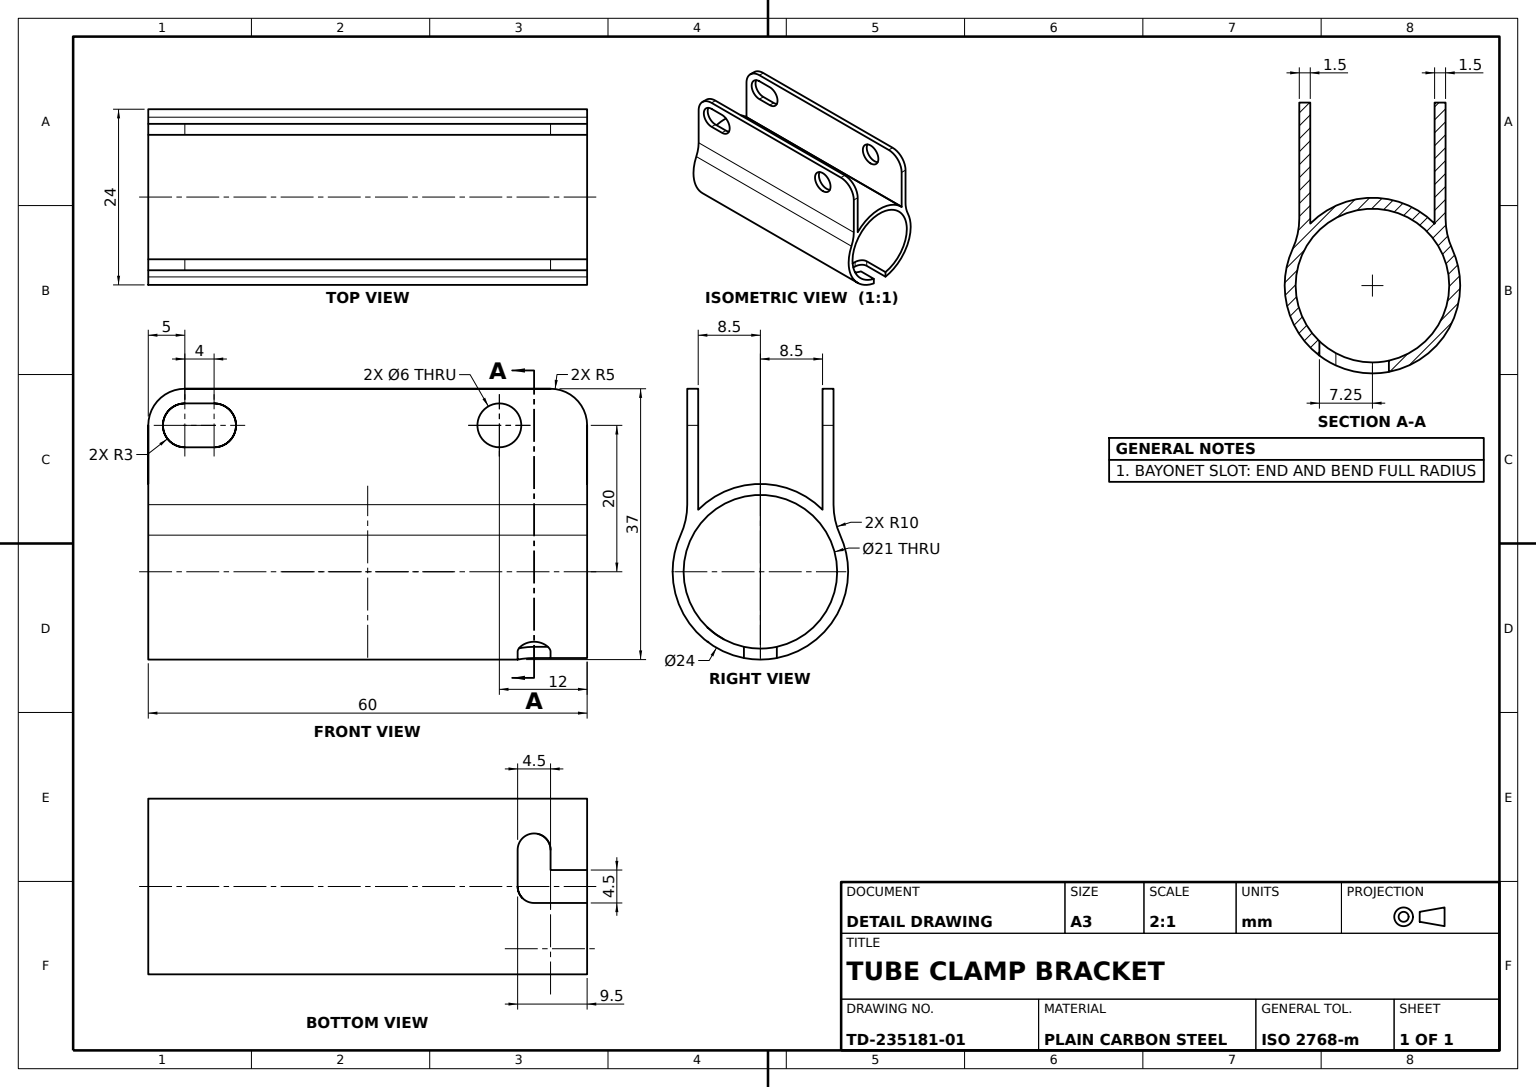
ISO-10303-21;
HEADER;
FILE_DESCRIPTION((''),'2;1');
FILE_NAME('','',(''),(''),'','','');
FILE_SCHEMA(('AUTOMOTIVE_DESIGN'));
ENDSEC;
DATA;
#1=APPLICATION_CONTEXT('');
#2=PRODUCT_CONTEXT('',#1,'mechanical');
#3=PRODUCT('','','',(#2));
#4=PRODUCT_DEFINITION_FORMATION('','',#3);
#5=PRODUCT_DEFINITION_CONTEXT('',#1,'design');
#6=PRODUCT_DEFINITION('','',#4,#5);
#7=PRODUCT_DEFINITION_SHAPE('','',#6);
#8=(LENGTH_UNIT()NAMED_UNIT(*)SI_UNIT(.MILLI.,.METRE.));
#9=(NAMED_UNIT(*)PLANE_ANGLE_UNIT()SI_UNIT($,.RADIAN.));
#10=(NAMED_UNIT(*)SI_UNIT($,.STERADIAN.)SOLID_ANGLE_UNIT());
#11=UNCERTAINTY_MEASURE_WITH_UNIT(LENGTH_MEASURE(1.E-05),#8,'distance_accuracy_value','');
#12=(GEOMETRIC_REPRESENTATION_CONTEXT(3)GLOBAL_UNCERTAINTY_ASSIGNED_CONTEXT((#11))GLOBAL_UNIT_ASSIGNED_CONTEXT((#8,#9,#10))REPRESENTATION_CONTEXT('',''));
#13=CARTESIAN_POINT('',(-10.909091,4.999173,30.));
#14=VERTEX_POINT('',#13);
#15=CARTESIAN_POINT('',(-10.909091,4.999173,-30.));
#16=VERTEX_POINT('',#15);
#17=DIRECTION('',(0.,0.,-1.));
#18=VECTOR('',#17,1000.);
#19=LINE('',#13,#18);
#20=EDGE_CURVE('',#14,#16,#19,.T.);
#21=ORIENTED_EDGE('',*,*,#20,.T.);
#22=CARTESIAN_POINT('',(-12.,0.,-30.));
#23=VERTEX_POINT('',#22);
#24=CARTESIAN_POINT('',(0.,0.,-30.));
#25=DIRECTION('',(0.,0.,1.));
#26=DIRECTION('',(1.,0.,0.));
#27=AXIS2_PLACEMENT_3D('',#24,#25,#26);
#28=CIRCLE('',#27,12.);
#29=EDGE_CURVE('',#16,#23,#28,.T.);
#30=ORIENTED_EDGE('',*,*,#29,.T.);
#31=CARTESIAN_POINT('',(-12.,0.,30.));
#32=VERTEX_POINT('',#31);
#33=LINE('',#31,#18);
#34=EDGE_CURVE('',#32,#23,#33,.T.);
#35=ORIENTED_EDGE('',*,*,#34,.F.);
#36=CARTESIAN_POINT('',(0.,0.,30.));
#37=AXIS2_PLACEMENT_3D('',#36,#25,#26);
#38=CIRCLE('',#37,12.);
#39=EDGE_CURVE('',#14,#32,#38,.T.);
#40=ORIENTED_EDGE('',*,*,#39,.F.);
#41=EDGE_LOOP('',(#21,#30,#35,#40));
#42=FACE_OUTER_BOUND('',#41,.T.);
#43=DIRECTION('',(-1.,0.,0.));
#44=AXIS2_PLACEMENT_3D('',#36,#17,#43);
#45=CYLINDRICAL_SURFACE('',#44,12.);
#46=ADVANCED_FACE('',(#42),#45,.T.);
#47=CARTESIAN_POINT('',(-2.25,-10.256096,-30.));
#48=VERTEX_POINT('',#47);
#49=CARTESIAN_POINT('',(-2.25,-10.256096,-22.75));
#50=VERTEX_POINT('',#49);
#51=CARTESIAN_POINT('',(-2.25,-10.256096,30.));
#52=VECTOR('',#25,1000.);
#53=LINE('',#51,#52);
#54=EDGE_CURVE('',#48,#50,#53,.T.);
#55=ORIENTED_EDGE('',*,*,#54,.T.);
#56=CARTESIAN_POINT('',(-2.25,-11.787175,-22.75));
#57=VERTEX_POINT('',#56);
#58=CARTESIAN_POINT('',(-2.25,-12.001,-22.75));
#59=DIRECTION('',(0.,1.,0.));
#60=VECTOR('',#59,1000.);
#61=LINE('',#58,#60);
#62=EDGE_CURVE('',#57,#50,#61,.T.);
#63=ORIENTED_EDGE('',*,*,#62,.F.);
#64=CARTESIAN_POINT('',(-2.25,-11.787175,-30.));
#65=VERTEX_POINT('',#64);
#66=CARTESIAN_POINT('',(-2.25,-11.787175,30.));
#67=LINE('',#66,#18);
#68=EDGE_CURVE('',#57,#65,#67,.T.);
#69=ORIENTED_EDGE('',*,*,#68,.T.);
#70=CARTESIAN_POINT('',(-2.25,-12.001,-30.));
#71=LINE('',#70,#60);
#72=EDGE_CURVE('',#65,#48,#71,.T.);
#73=ORIENTED_EDGE('',*,*,#72,.T.);
#74=EDGE_LOOP('',(#55,#63,#69,#73));
#75=FACE_OUTER_BOUND('',#74,.T.);
#76=AXIS2_PLACEMENT_3D('',#70,#43,#25);
#77=PLANE('',#76);
#78=ADVANCED_FACE('',(#75),#77,.F.);
#79=CARTESIAN_POINT('',(10.909091,4.999173,30.));
#80=VERTEX_POINT('',#79);
#81=CARTESIAN_POINT('',(10.,9.165151,30.));
#82=VERTEX_POINT('',#81);
#83=CARTESIAN_POINT('',(20.,9.165151,30.));
#84=AXIS2_PLACEMENT_3D('',#83,#17,#26);
#85=CIRCLE('',#84,10.);
#86=EDGE_CURVE('',#80,#82,#85,.T.);
#87=ORIENTED_EDGE('',*,*,#86,.F.);
#88=CARTESIAN_POINT('',(10.909091,4.999173,-30.));
#89=VERTEX_POINT('',#88);
#90=LINE('',#79,#52);
#91=EDGE_CURVE('',#89,#80,#90,.T.);
#92=ORIENTED_EDGE('',*,*,#91,.F.);
#93=CARTESIAN_POINT('',(10.,9.165151,-30.));
#94=VERTEX_POINT('',#93);
#95=CARTESIAN_POINT('',(20.,9.165151,-30.));
#96=AXIS2_PLACEMENT_3D('',#95,#25,#26);
#97=CIRCLE('',#96,10.);
#98=EDGE_CURVE('',#94,#89,#97,.T.);
#99=ORIENTED_EDGE('',*,*,#98,.F.);
#100=LINE('',#93,#18);
#101=EDGE_CURVE('',#82,#94,#100,.T.);
#102=ORIENTED_EDGE('',*,*,#101,.F.);
#103=EDGE_LOOP('',(#87,#92,#99,#102));
#104=FACE_OUTER_BOUND('',#103,.T.);
#105=AXIS2_PLACEMENT_3D('',#83,#17,#43);
#106=CYLINDRICAL_SURFACE('',#105,10.);
#107=ADVANCED_FACE('',(#104),#106,.F.);
#108=CARTESIAN_POINT('',(12.,0.,30.));
#109=VERTEX_POINT('',#108);
#110=EDGE_CURVE('',#109,#80,#38,.T.);
#111=ORIENTED_EDGE('',*,*,#110,.F.);
#112=CARTESIAN_POINT('',(12.,0.,-30.));
#113=VERTEX_POINT('',#112);
#114=LINE('',#108,#18);
#115=EDGE_CURVE('',#109,#113,#114,.T.);
#116=ORIENTED_EDGE('',*,*,#115,.T.);
#117=EDGE_CURVE('',#113,#89,#28,.T.);
#118=ORIENTED_EDGE('',*,*,#117,.T.);
#119=ORIENTED_EDGE('',*,*,#91,.T.);
#120=EDGE_LOOP('',(#111,#116,#118,#119));
#121=FACE_OUTER_BOUND('',#120,.T.);
#122=ADVANCED_FACE('',(#121),#45,.T.);
#123=CARTESIAN_POINT('',(2.25,-11.787175,-25.));
#124=VERTEX_POINT('',#123);
#125=CARTESIAN_POINT('',(5.,-10.908712,-25.));
#126=VERTEX_POINT('',#125);
#127=CARTESIAN_POINT('',(0.,0.,-25.));
#128=AXIS2_PLACEMENT_3D('',#127,#25,#43);
#129=CIRCLE('',#128,12.);
#130=EDGE_CURVE('',#124,#126,#129,.T.);
#131=ORIENTED_EDGE('',*,*,#130,.F.);
#132=CARTESIAN_POINT('',(2.25,-11.787175,-30.));
#133=VERTEX_POINT('',#132);
#134=CARTESIAN_POINT('',(2.25,-11.787175,30.));
#135=LINE('',#134,#52);
#136=EDGE_CURVE('',#133,#124,#135,.T.);
#137=ORIENTED_EDGE('',*,*,#136,.F.);
#138=EDGE_CURVE('',#133,#113,#28,.T.);
#139=ORIENTED_EDGE('',*,*,#138,.T.);
#140=ORIENTED_EDGE('',*,*,#115,.F.);
#141=EDGE_CURVE('',#32,#109,#38,.T.);
#142=ORIENTED_EDGE('',*,*,#141,.F.);
#143=ORIENTED_EDGE('',*,*,#34,.T.);
#144=EDGE_CURVE('',#23,#65,#28,.T.);
#145=ORIENTED_EDGE('',*,*,#144,.T.);
#146=ORIENTED_EDGE('',*,*,#68,.F.);
#147=CARTESIAN_POINT('',(0.,-12.,-20.5));
#148=VERTEX_POINT('',#147);
#149=CARTESIAN_POINT('',(-0.148916,-12.,-20.5));
#150=CARTESIAN_POINT('',(-0.29528,-11.997231,-20.514638));
#151=CARTESIAN_POINT('',(-0.583133,-11.986688,-20.571929));
#152=CARTESIAN_POINT('',(-0.726135,-11.978787,-20.615301));
#153=CARTESIAN_POINT('',(-0.998336,-11.959178,-20.728234));
#154=CARTESIAN_POINT('',(-1.127389,-11.947555,-20.797295));
#155=CARTESIAN_POINT('',(-1.371629,-11.921984,-20.960392));
#156=CARTESIAN_POINT('',(-1.487027,-11.907966,-21.055107));
#157=CARTESIAN_POINT('',(-1.797526,-11.866445,-21.365425));
#158=CARTESIAN_POINT('',(-1.965077,-11.83856,-21.615671));
#159=CARTESIAN_POINT('',(-2.189941,-11.799033,-22.156375));
#160=CARTESIAN_POINT('',(-2.25,-11.787175,-22.452172));
#161=B_SPLINE_CURVE_WITH_KNOTS('',3,(#147,#149,#150,#151,#152,#153,#154,#155,#156,#157,#158,#159,#160,#56),.UNSPECIFIED.,.F.,.F.,(4,2,2,2,2,2,4),(0.,0.000440334,0.000880667,0.001321001,0.001761334,0.002642001,0.003522668),.UNSPECIFIED.);
#162=EDGE_CURVE('',#148,#57,#161,.T.);
#163=ORIENTED_EDGE('',*,*,#162,.F.);
#164=CARTESIAN_POINT('',(5.,-10.908712,-20.5));
#165=VERTEX_POINT('',#164);
#166=CARTESIAN_POINT('',(0.,0.,-20.5));
#167=AXIS2_PLACEMENT_3D('',#166,#17,#26);
#168=CIRCLE('',#167,12.);
#169=EDGE_CURVE('',#165,#148,#168,.T.);
#170=ORIENTED_EDGE('',*,*,#169,.F.);
#171=CARTESIAN_POINT('',(5.291277,-10.775206,-25.));
#172=CARTESIAN_POINT('',(5.568793,-10.633901,-24.945399));
#173=CARTESIAN_POINT('',(6.096925,-10.340155,-24.734958));
#174=CARTESIAN_POINT('',(6.334777,-10.194776,-24.584238));
#175=CARTESIAN_POINT('',(6.755082,-9.921277,-24.187271));
#176=CARTESIAN_POINT('',(6.927005,-9.800041,-23.951534));
#177=CARTESIAN_POINT('',(7.115788,-9.662899,-23.530752));
#178=CARTESIAN_POINT('',(7.164502,-9.626613,-23.384151));
#179=CARTESIAN_POINT('',(7.23166,-9.576265,-23.076973));
#180=CARTESIAN_POINT('',(7.24941,-9.562743,-22.916453));
#181=CARTESIAN_POINT('',(7.250561,-9.561871,-22.599906));
#182=CARTESIAN_POINT('',(7.233989,-9.5745,-22.439219));
#183=CARTESIAN_POINT('',(7.168929,-9.623311,-22.131097));
#184=CARTESIAN_POINT('',(7.120922,-9.659108,-21.983251));
#185=CARTESIAN_POINT('',(6.996677,-9.749482,-21.701433));
#186=CARTESIAN_POINT('',(6.922276,-9.8027,-21.571326));
#187=CARTESIAN_POINT('',(6.751271,-9.921248,-21.329625));
#188=CARTESIAN_POINT('',(6.654513,-9.986635,-21.218426));
#189=CARTESIAN_POINT('',(6.342224,-10.19009,-20.921485));
#190=CARTESIAN_POINT('',(6.098757,-10.338984,-20.766451));
#191=CARTESIAN_POINT('',(5.576237,-10.629911,-20.5569));
#192=CARTESIAN_POINT('',(5.291702,-10.775011,-20.5));
#193=B_SPLINE_CURVE_WITH_KNOTS('',3,(#125,#171,#172,#173,#174,#175,#176,#177,#178,#179,#180,#181,#182,#183,#184,#185,#186,#187,#188,#189,#190,#191,#192,#164),.UNSPECIFIED.,.F.,.F.,(4,2,2,2,2,2,2,2,2,2,2,4),(0.,0.000947115,0.001894231,0.002841346,0.003314904,0.003788462,0.004262019,0.004735577,0.005209135,0.005682693,0.006629808,0.007576923),.UNSPECIFIED.);
#194=EDGE_CURVE('',#126,#165,#193,.T.);
#195=ORIENTED_EDGE('',*,*,#194,.F.);
#196=EDGE_LOOP('',(#131,#137,#139,#140,#142,#143,#145,#146,#163,#170,#195));
#197=FACE_OUTER_BOUND('',#196,.T.);
#198=ADVANCED_FACE('',(#197),#45,.T.);
#199=CARTESIAN_POINT('',(-10.,20.,-30.));
#200=VERTEX_POINT('',#199);
#201=CARTESIAN_POINT('',(-8.5,20.,-30.));
#202=VERTEX_POINT('',#201);
#203=VECTOR('',#26,1000.);
#204=LINE('',#201,#203);
#205=EDGE_CURVE('',#200,#202,#204,.T.);
#206=ORIENTED_EDGE('',*,*,#205,.F.);
#207=CARTESIAN_POINT('',(-10.,25.,-25.));
#208=VERTEX_POINT('',#207);
#209=CARTESIAN_POINT('',(-10.,20.,-25.));
#210=DIRECTION('',(0.,-1.,0.));
#211=AXIS2_PLACEMENT_3D('',#209,#43,#210);
#212=CIRCLE('',#211,5.);
#213=EDGE_CURVE('',#208,#200,#212,.T.);
#214=ORIENTED_EDGE('',*,*,#213,.F.);
#215=CARTESIAN_POINT('',(-8.5,25.,-25.));
#216=VERTEX_POINT('',#215);
#217=VECTOR('',#43,1000.);
#218=LINE('',#207,#217);
#219=EDGE_CURVE('',#216,#208,#218,.T.);
#220=ORIENTED_EDGE('',*,*,#219,.F.);
#221=CARTESIAN_POINT('',(-8.5,20.,-25.));
#222=AXIS2_PLACEMENT_3D('',#221,#26,#59);
#223=CIRCLE('',#222,5.);
#224=EDGE_CURVE('',#202,#216,#223,.T.);
#225=ORIENTED_EDGE('',*,*,#224,.F.);
#226=EDGE_LOOP('',(#206,#214,#220,#225));
#227=FACE_OUTER_BOUND('',#226,.T.);
#228=AXIS2_PLACEMENT_3D('',#209,#26,#17);
#229=CYLINDRICAL_SURFACE('',#228,5.);
#230=ADVANCED_FACE('',(#227),#229,.T.);
#231=CARTESIAN_POINT('',(8.5,20.,-30.));
#232=VERTEX_POINT('',#231);
#233=CARTESIAN_POINT('',(10.,20.,-30.));
#234=VERTEX_POINT('',#233);
#235=LINE('',#233,#203);
#236=EDGE_CURVE('',#232,#234,#235,.T.);
#237=ORIENTED_EDGE('',*,*,#236,.F.);
#238=CARTESIAN_POINT('',(8.5,25.,-25.));
#239=VERTEX_POINT('',#238);
#240=CARTESIAN_POINT('',(8.5,20.,-25.));
#241=AXIS2_PLACEMENT_3D('',#240,#43,#210);
#242=CIRCLE('',#241,5.);
#243=EDGE_CURVE('',#239,#232,#242,.T.);
#244=ORIENTED_EDGE('',*,*,#243,.F.);
#245=CARTESIAN_POINT('',(10.,25.,-25.));
#246=VERTEX_POINT('',#245);
#247=LINE('',#238,#217);
#248=EDGE_CURVE('',#246,#239,#247,.T.);
#249=ORIENTED_EDGE('',*,*,#248,.F.);
#250=CARTESIAN_POINT('',(10.,20.,-25.));
#251=AXIS2_PLACEMENT_3D('',#250,#26,#59);
#252=CIRCLE('',#251,5.);
#253=EDGE_CURVE('',#234,#246,#252,.T.);
#254=ORIENTED_EDGE('',*,*,#253,.F.);
#255=EDGE_LOOP('',(#237,#244,#249,#254));
#256=FACE_OUTER_BOUND('',#255,.T.);
#257=AXIS2_PLACEMENT_3D('',#250,#26,#17);
#258=CYLINDRICAL_SURFACE('',#257,5.);
#259=ADVANCED_FACE('',(#256),#258,.T.);
#260=CARTESIAN_POINT('',(-10.,9.165151,-30.));
#261=VERTEX_POINT('',#260);
#262=CARTESIAN_POINT('',(-10.,9.165151,30.));
#263=VERTEX_POINT('',#262);
#264=LINE('',#260,#52);
#265=EDGE_CURVE('',#261,#263,#264,.T.);
#266=ORIENTED_EDGE('',*,*,#265,.F.);
#267=CARTESIAN_POINT('',(-20.,9.165151,-30.));
#268=AXIS2_PLACEMENT_3D('',#267,#25,#26);
#269=CIRCLE('',#268,10.);
#270=EDGE_CURVE('',#16,#261,#269,.T.);
#271=ORIENTED_EDGE('',*,*,#270,.F.);
#272=ORIENTED_EDGE('',*,*,#20,.F.);
#273=CARTESIAN_POINT('',(-20.,9.165151,30.));
#274=AXIS2_PLACEMENT_3D('',#273,#17,#26);
#275=CIRCLE('',#274,10.);
#276=EDGE_CURVE('',#263,#14,#275,.T.);
#277=ORIENTED_EDGE('',*,*,#276,.F.);
#278=EDGE_LOOP('',(#266,#271,#272,#277));
#279=FACE_OUTER_BOUND('',#278,.T.);
#280=AXIS2_PLACEMENT_3D('',#273,#17,#43);
#281=CYLINDRICAL_SURFACE('',#280,10.);
#282=ADVANCED_FACE('',(#279),#281,.F.);
#283=CARTESIAN_POINT('',(5.,-9.233093,-20.5));
#284=VERTEX_POINT('',#283);
#285=CARTESIAN_POINT('',(5.,-12.001,-20.5));
#286=LINE('',#285,#60);
#287=EDGE_CURVE('',#165,#284,#286,.T.);
#288=ORIENTED_EDGE('',*,*,#287,.F.);
#289=ORIENTED_EDGE('',*,*,#169,.T.);
#290=CARTESIAN_POINT('',(0.,-10.5,-20.5));
#291=VERTEX_POINT('',#290);
#292=CARTESIAN_POINT('',(0.,-12.001,-20.5));
#293=LINE('',#292,#60);
#294=EDGE_CURVE('',#148,#291,#293,.T.);
#295=ORIENTED_EDGE('',*,*,#294,.T.);
#296=AXIS2_PLACEMENT_3D('',#166,#25,#26);
#297=CIRCLE('',#296,10.5);
#298=EDGE_CURVE('',#291,#284,#297,.T.);
#299=ORIENTED_EDGE('',*,*,#298,.T.);
#300=EDGE_LOOP('',(#288,#289,#295,#299));
#301=FACE_OUTER_BOUND('',#300,.T.);
#302=AXIS2_PLACEMENT_3D('',#292,#25,#26);
#303=PLANE('',#302);
#304=ADVANCED_FACE('',(#301),#303,.F.);
#305=CARTESIAN_POINT('',(-10.,25.,-30.));
#306=VECTOR('',#210,1000.);
#307=LINE('',#305,#306);
#308=EDGE_CURVE('',#200,#261,#307,.T.);
#309=ORIENTED_EDGE('',*,*,#308,.F.);
#310=ORIENTED_EDGE('',*,*,#205,.T.);
#311=CARTESIAN_POINT('',(-8.5,8.470537,-30.));
#312=VERTEX_POINT('',#311);
#313=CARTESIAN_POINT('',(-8.5,25.,-30.));
#314=LINE('',#313,#60);
#315=EDGE_CURVE('',#312,#202,#314,.T.);
#316=ORIENTED_EDGE('',*,*,#315,.F.);
#317=CARTESIAN_POINT('',(8.5,8.470537,-30.));
#318=VERTEX_POINT('',#317);
#319=EDGE_CURVE('',#318,#312,#28,.T.);
#320=ORIENTED_EDGE('',*,*,#319,.F.);
#321=CARTESIAN_POINT('',(8.5,25.,-30.));
#322=LINE('',#321,#306);
#323=EDGE_CURVE('',#232,#318,#322,.T.);
#324=ORIENTED_EDGE('',*,*,#323,.F.);
#325=ORIENTED_EDGE('',*,*,#236,.T.);
#326=CARTESIAN_POINT('',(10.,25.,-30.));
#327=LINE('',#326,#60);
#328=EDGE_CURVE('',#94,#234,#327,.T.);
#329=ORIENTED_EDGE('',*,*,#328,.F.);
#330=ORIENTED_EDGE('',*,*,#98,.T.);
#331=ORIENTED_EDGE('',*,*,#117,.F.);
#332=ORIENTED_EDGE('',*,*,#138,.F.);
#333=CARTESIAN_POINT('',(2.25,-10.256096,-30.));
#334=VERTEX_POINT('',#333);
#335=CARTESIAN_POINT('',(2.25,-12.001,-30.));
#336=LINE('',#335,#60);
#337=EDGE_CURVE('',#133,#334,#336,.T.);
#338=ORIENTED_EDGE('',*,*,#337,.T.);
#339=CARTESIAN_POINT('',(10.5,0.,-30.));
#340=VERTEX_POINT('',#339);
#341=CIRCLE('',#27,10.5);
#342=EDGE_CURVE('',#334,#340,#341,.T.);
#343=ORIENTED_EDGE('',*,*,#342,.T.);
#344=CARTESIAN_POINT('',(-10.5,0.,-30.));
#345=VERTEX_POINT('',#344);
#346=EDGE_CURVE('',#340,#345,#341,.T.);
#347=ORIENTED_EDGE('',*,*,#346,.T.);
#348=EDGE_CURVE('',#345,#48,#341,.T.);
#349=ORIENTED_EDGE('',*,*,#348,.T.);
#350=ORIENTED_EDGE('',*,*,#72,.F.);
#351=ORIENTED_EDGE('',*,*,#144,.F.);
#352=ORIENTED_EDGE('',*,*,#29,.F.);
#353=ORIENTED_EDGE('',*,*,#270,.T.);
#354=EDGE_LOOP('',(#309,#310,#316,#320,#324,#325,#329,#330,#331,#332,#338,#343,#347,#349,#350,#351,#352,#353));
#355=FACE_OUTER_BOUND('',#354,.T.);
#356=PLANE('',#27);
#357=ADVANCED_FACE('',(#355),#356,.F.);
#358=ORIENTED_EDGE('',*,*,#319,.T.);
#359=CARTESIAN_POINT('',(-8.5,8.470537,30.));
#360=VERTEX_POINT('',#359);
#361=LINE('',#311,#52);
#362=EDGE_CURVE('',#312,#360,#361,.T.);
#363=ORIENTED_EDGE('',*,*,#362,.T.);
#364=CARTESIAN_POINT('',(8.5,8.470537,30.));
#365=VERTEX_POINT('',#364);
#366=EDGE_CURVE('',#365,#360,#38,.T.);
#367=ORIENTED_EDGE('',*,*,#366,.F.);
#368=LINE('',#317,#52);
#369=EDGE_CURVE('',#318,#365,#368,.T.);
#370=ORIENTED_EDGE('',*,*,#369,.F.);
#371=EDGE_LOOP('',(#358,#363,#367,#370));
#372=FACE_OUTER_BOUND('',#371,.T.);
#373=ADVANCED_FACE('',(#372),#45,.T.);
#374=CARTESIAN_POINT('',(-10.,17.,-18.));
#375=VERTEX_POINT('',#374);
#376=CARTESIAN_POINT('',(-10.,23.,-18.));
#377=VERTEX_POINT('',#376);
#378=CARTESIAN_POINT('',(-10.,20.,-18.));
#379=AXIS2_PLACEMENT_3D('',#378,#43,#210);
#380=CIRCLE('',#379,3.);
#381=EDGE_CURVE('',#375,#377,#380,.T.);
#382=ORIENTED_EDGE('',*,*,#381,.F.);
#383=EDGE_CURVE('',#377,#375,#380,.T.);
#384=ORIENTED_EDGE('',*,*,#383,.F.);
#385=EDGE_LOOP('',(#382,#384));
#386=FACE_BOUND('',#385,.T.);
#387=ORIENTED_EDGE('',*,*,#265,.T.);
#388=CARTESIAN_POINT('',(-10.,20.,30.));
#389=VERTEX_POINT('',#388);
#390=CARTESIAN_POINT('',(-10.,25.,30.));
#391=LINE('',#390,#306);
#392=EDGE_CURVE('',#389,#263,#391,.T.);
#393=ORIENTED_EDGE('',*,*,#392,.F.);
#394=CARTESIAN_POINT('',(-10.,25.,25.));
#395=VERTEX_POINT('',#394);
#396=CARTESIAN_POINT('',(-10.,20.,25.));
#397=AXIS2_PLACEMENT_3D('',#396,#43,#210);
#398=CIRCLE('',#397,5.);
#399=EDGE_CURVE('',#389,#395,#398,.T.);
#400=ORIENTED_EDGE('',*,*,#399,.T.);
#401=LINE('',#305,#52);
#402=EDGE_CURVE('',#208,#395,#401,.T.);
#403=ORIENTED_EDGE('',*,*,#402,.F.);
#404=ORIENTED_EDGE('',*,*,#213,.T.);
#405=ORIENTED_EDGE('',*,*,#308,.T.);
#406=EDGE_LOOP('',(#387,#393,#400,#403,#404,#405));
#407=FACE_OUTER_BOUND('',#406,.T.);
#408=CARTESIAN_POINT('',(-10.,17.,25.));
#409=VERTEX_POINT('',#408);
#410=CARTESIAN_POINT('',(-10.,23.,25.));
#411=VERTEX_POINT('',#410);
#412=CIRCLE('',#397,3.);
#413=EDGE_CURVE('',#409,#411,#412,.T.);
#414=ORIENTED_EDGE('',*,*,#413,.F.);
#415=CARTESIAN_POINT('',(-10.,17.,21.));
#416=VERTEX_POINT('',#415);
#417=CARTESIAN_POINT('',(-10.,17.,-30.));
#418=LINE('',#417,#52);
#419=EDGE_CURVE('',#416,#409,#418,.T.);
#420=ORIENTED_EDGE('',*,*,#419,.F.);
#421=CARTESIAN_POINT('',(-10.,23.,21.));
#422=VERTEX_POINT('',#421);
#423=CARTESIAN_POINT('',(-10.,20.,21.));
#424=AXIS2_PLACEMENT_3D('',#423,#43,#210);
#425=CIRCLE('',#424,3.);
#426=EDGE_CURVE('',#422,#416,#425,.T.);
#427=ORIENTED_EDGE('',*,*,#426,.F.);
#428=CARTESIAN_POINT('',(-10.,23.,-30.));
#429=LINE('',#428,#18);
#430=EDGE_CURVE('',#411,#422,#429,.T.);
#431=ORIENTED_EDGE('',*,*,#430,.F.);
#432=EDGE_LOOP('',(#414,#420,#427,#431));
#433=FACE_BOUND('',#432,.T.);
#434=AXIS2_PLACEMENT_3D('',#305,#43,#210);
#435=PLANE('',#434);
#436=ADVANCED_FACE('',(#386,#407,#433),#435,.T.);
#437=CARTESIAN_POINT('',(10.5,0.,30.));
#438=VERTEX_POINT('',#437);
#439=CARTESIAN_POINT('',(-10.5,0.,30.));
#440=VERTEX_POINT('',#439);
#441=CIRCLE('',#37,10.5);
#442=EDGE_CURVE('',#438,#440,#441,.T.);
#443=ORIENTED_EDGE('',*,*,#442,.T.);
#444=LINE('',#439,#18);
#445=EDGE_CURVE('',#440,#345,#444,.T.);
#446=ORIENTED_EDGE('',*,*,#445,.T.);
#447=ORIENTED_EDGE('',*,*,#346,.F.);
#448=LINE('',#437,#18);
#449=EDGE_CURVE('',#438,#340,#448,.T.);
#450=ORIENTED_EDGE('',*,*,#449,.F.);
#451=EDGE_LOOP('',(#443,#446,#447,#450));
#452=FACE_OUTER_BOUND('',#451,.T.);
#453=CYLINDRICAL_SURFACE('',#44,10.5);
#454=ADVANCED_FACE('',(#452),#453,.F.);
#455=EDGE_CURVE('',#440,#438,#441,.T.);
#456=ORIENTED_EDGE('',*,*,#455,.F.);
#457=ORIENTED_EDGE('',*,*,#442,.F.);
#458=EDGE_LOOP('',(#456,#457));
#459=FACE_BOUND('',#458,.T.);
#460=CARTESIAN_POINT('',(-8.5,20.,30.));
#461=VERTEX_POINT('',#460);
#462=CARTESIAN_POINT('',(-8.5,25.,30.));
#463=LINE('',#462,#60);
#464=EDGE_CURVE('',#360,#461,#463,.T.);
#465=ORIENTED_EDGE('',*,*,#464,.T.);
#466=CARTESIAN_POINT('',(0.,20.,30.));
#467=LINE('',#466,#217);
#468=EDGE_CURVE('',#461,#389,#467,.T.);
#469=ORIENTED_EDGE('',*,*,#468,.T.);
#470=ORIENTED_EDGE('',*,*,#392,.T.);
#471=ORIENTED_EDGE('',*,*,#276,.T.);
#472=ORIENTED_EDGE('',*,*,#39,.T.);
#473=ORIENTED_EDGE('',*,*,#141,.T.);
#474=ORIENTED_EDGE('',*,*,#110,.T.);
#475=ORIENTED_EDGE('',*,*,#86,.T.);
#476=CARTESIAN_POINT('',(10.,20.,30.));
#477=VERTEX_POINT('',#476);
#478=CARTESIAN_POINT('',(10.,25.,30.));
#479=LINE('',#478,#60);
#480=EDGE_CURVE('',#82,#477,#479,.T.);
#481=ORIENTED_EDGE('',*,*,#480,.T.);
#482=CARTESIAN_POINT('',(8.5,20.,30.));
#483=VERTEX_POINT('',#482);
#484=EDGE_CURVE('',#477,#483,#467,.T.);
#485=ORIENTED_EDGE('',*,*,#484,.T.);
#486=CARTESIAN_POINT('',(8.5,25.,30.));
#487=LINE('',#486,#306);
#488=EDGE_CURVE('',#483,#365,#487,.T.);
#489=ORIENTED_EDGE('',*,*,#488,.T.);
#490=ORIENTED_EDGE('',*,*,#366,.T.);
#491=EDGE_LOOP('',(#465,#469,#470,#471,#472,#473,#474,#475,#481,#485,#489,#490));
#492=FACE_OUTER_BOUND('',#491,.T.);
#493=PLANE('',#37);
#494=ADVANCED_FACE('',(#459,#492),#493,.T.);
#495=ORIENTED_EDGE('',*,*,#337,.F.);
#496=ORIENTED_EDGE('',*,*,#136,.T.);
#497=CARTESIAN_POINT('',(2.25,-10.256096,-25.));
#498=VERTEX_POINT('',#497);
#499=CARTESIAN_POINT('',(2.25,-12.001,-25.));
#500=LINE('',#499,#60);
#501=EDGE_CURVE('',#124,#498,#500,.T.);
#502=ORIENTED_EDGE('',*,*,#501,.T.);
#503=CARTESIAN_POINT('',(2.25,-10.256096,30.));
#504=LINE('',#503,#18);
#505=EDGE_CURVE('',#498,#334,#504,.T.);
#506=ORIENTED_EDGE('',*,*,#505,.T.);
#507=EDGE_LOOP('',(#495,#496,#502,#506));
#508=FACE_OUTER_BOUND('',#507,.T.);
#509=AXIS2_PLACEMENT_3D('',#499,#26,#17);
#510=PLANE('',#509);
#511=ADVANCED_FACE('',(#508),#510,.F.);
#512=CARTESIAN_POINT('',(5.,-9.233093,-25.));
#513=VERTEX_POINT('',#512);
#514=CARTESIAN_POINT('',(5.291373,-9.075305,-20.5));
#515=CARTESIAN_POINT('',(5.565419,-8.909164,-20.55445));
#516=CARTESIAN_POINT('',(5.954291,-8.649895,-20.707639));
#517=CARTESIAN_POINT('',(6.08017,-8.561705,-20.771347));
#518=CARTESIAN_POINT('',(6.315583,-8.389557,-20.919405));
#519=CARTESIAN_POINT('',(6.426392,-8.304764,-21.004146));
#520=CARTESIAN_POINT('',(6.634249,-8.139678,-21.196993));
#521=CARTESIAN_POINT('',(6.731534,-8.059114,-21.305802));
#522=CARTESIAN_POINT('',(6.904028,-7.911843,-21.542276));
#523=CARTESIAN_POINT('',(6.980308,-7.844293,-21.670645));
#524=CARTESIAN_POINT('',(7.109836,-7.727086,-21.952995));
#525=CARTESIAN_POINT('',(7.160609,-7.679714,-22.101687));
#526=CARTESIAN_POINT('',(7.231015,-7.613459,-22.416664));
#527=CARTESIAN_POINT('',(7.249658,-7.595555,-22.581838));
#528=CARTESIAN_POINT('',(7.250332,-7.594911,-22.908881));
#529=CARTESIAN_POINT('',(7.232158,-7.612368,-23.075443));
#530=CARTESIAN_POINT('',(7.163042,-7.67744,-23.390071));
#531=CARTESIAN_POINT('',(7.111547,-7.725497,-23.542169));
#532=CARTESIAN_POINT('',(6.920363,-7.898617,-23.962168));
#533=CARTESIAN_POINT('',(6.742094,-8.053803,-24.201687));
#534=CARTESIAN_POINT('',(6.329198,-8.382173,-24.587259));
#535=CARTESIAN_POINT('',(6.088851,-8.55992,-24.73848));
#536=CARTESIAN_POINT('',(5.572584,-8.904642,-24.943581));
#537=CARTESIAN_POINT('',(5.291164,-9.075419,-25.));
#538=B_SPLINE_CURVE_WITH_KNOTS('',3,(#283,#514,#515,#516,#517,#518,#519,#520,#521,#522,#523,#524,#525,#526,#527,#528,#529,#530,#531,#532,#533,#534,#535,#536,#537,#512),.UNSPECIFIED.,.F.,.F.,(4,2,2,2,2,2,2,2,2,2,2,2,4),(0.,0.000974985,0.001462477,0.00194997,0.002437462,0.002924955,0.003412447,0.00389994,0.004387432,0.004874924,0.005849909,0.006824894,0.007799879),.UNSPECIFIED.);
#539=EDGE_CURVE('',#284,#513,#538,.T.);
#540=ORIENTED_EDGE('',*,*,#539,.T.);
#541=CARTESIAN_POINT('',(5.,-12.001,-25.));
#542=LINE('',#541,#60);
#543=EDGE_CURVE('',#126,#513,#542,.T.);
#544=ORIENTED_EDGE('',*,*,#543,.F.);
#545=ORIENTED_EDGE('',*,*,#194,.T.);
#546=ORIENTED_EDGE('',*,*,#287,.T.);
#547=EDGE_LOOP('',(#540,#544,#545,#546));
#548=FACE_OUTER_BOUND('',#547,.T.);
#549=CARTESIAN_POINT('',(5.,-12.001,-22.75));
#550=AXIS2_PLACEMENT_3D('',#549,#59,#25);
#551=CYLINDRICAL_SURFACE('',#550,2.25);
#552=ADVANCED_FACE('',(#548),#551,.F.);
#553=CARTESIAN_POINT('',(-8.5,23.,25.));
#554=VERTEX_POINT('',#553);
#555=CARTESIAN_POINT('',(-50.,23.,25.));
#556=LINE('',#555,#203);
#557=EDGE_CURVE('',#411,#554,#556,.T.);
#558=ORIENTED_EDGE('',*,*,#557,.T.);
#559=CARTESIAN_POINT('',(-8.5,17.,25.));
#560=VERTEX_POINT('',#559);
#561=CARTESIAN_POINT('',(-8.5,20.,25.));
#562=AXIS2_PLACEMENT_3D('',#561,#26,#59);
#563=CIRCLE('',#562,3.);
#564=EDGE_CURVE('',#554,#560,#563,.T.);
#565=ORIENTED_EDGE('',*,*,#564,.T.);
#566=CARTESIAN_POINT('',(-50.,17.,25.));
#567=LINE('',#566,#203);
#568=EDGE_CURVE('',#409,#560,#567,.T.);
#569=ORIENTED_EDGE('',*,*,#568,.F.);
#570=ORIENTED_EDGE('',*,*,#413,.T.);
#571=EDGE_LOOP('',(#558,#565,#569,#570));
#572=FACE_OUTER_BOUND('',#571,.T.);
#573=CARTESIAN_POINT('',(-50.,20.,25.));
#574=AXIS2_PLACEMENT_3D('',#573,#26,#59);
#575=CYLINDRICAL_SURFACE('',#574,3.);
#576=ADVANCED_FACE('',(#572),#575,.F.);
#577=CARTESIAN_POINT('',(-2.25,-10.256096,-22.600971));
#578=CARTESIAN_POINT('',(-2.235341,-10.259343,-22.454521));
#579=CARTESIAN_POINT('',(-2.177987,-10.271671,-22.166537));
#580=CARTESIAN_POINT('',(-2.134567,-10.280902,-22.023484));
#581=CARTESIAN_POINT('',(-2.02161,-10.303709,-21.751352));
#582=CARTESIAN_POINT('',(-1.952551,-10.31719,-21.622349));
#583=CARTESIAN_POINT('',(-1.789469,-10.346722,-21.378194));
#584=CARTESIAN_POINT('',(-1.69484,-10.36284,-21.262924));
#585=CARTESIAN_POINT('',(-1.384772,-10.410386,-20.952663));
#586=CARTESIAN_POINT('',(-1.134677,-10.442035,-20.785124));
#587=CARTESIAN_POINT('',(-0.594021,-10.486692,-20.560167));
#588=CARTESIAN_POINT('',(-0.298047,-10.5,-20.5));
#589=B_SPLINE_CURVE_WITH_KNOTS('',3,(#49,#577,#578,#579,#580,#581,#582,#583,#584,#585,#586,#587,#588,#290),.UNSPECIFIED.,.F.,.F.,(4,2,2,2,2,2,4),(0.,0.000440637,0.000881274,0.001321911,0.001762547,0.002643821,0.003525095),.UNSPECIFIED.);
#590=EDGE_CURVE('',#50,#291,#589,.T.);
#591=ORIENTED_EDGE('',*,*,#590,.T.);
#592=ORIENTED_EDGE('',*,*,#294,.F.);
#593=ORIENTED_EDGE('',*,*,#162,.T.);
#594=ORIENTED_EDGE('',*,*,#62,.T.);
#595=EDGE_LOOP('',(#591,#592,#593,#594));
#596=FACE_OUTER_BOUND('',#595,.T.);
#597=CARTESIAN_POINT('',(0.,-12.001,-22.75));
#598=AXIS2_PLACEMENT_3D('',#597,#59,#25);
#599=CYLINDRICAL_SURFACE('',#598,2.25);
#600=ADVANCED_FACE('',(#596),#599,.F.);
#601=CARTESIAN_POINT('',(8.5,23.,21.));
#602=VERTEX_POINT('',#601);
#603=CARTESIAN_POINT('',(10.,23.,21.));
#604=VERTEX_POINT('',#603);
#605=CARTESIAN_POINT('',(-50.,23.,21.));
#606=LINE('',#605,#203);
#607=EDGE_CURVE('',#602,#604,#606,.T.);
#608=ORIENTED_EDGE('',*,*,#607,.T.);
#609=CARTESIAN_POINT('',(10.,23.,25.));
#610=VERTEX_POINT('',#609);
#611=LINE('',#609,#52);
#612=EDGE_CURVE('',#604,#610,#611,.T.);
#613=ORIENTED_EDGE('',*,*,#612,.T.);
#614=CARTESIAN_POINT('',(8.5,23.,25.));
#615=VERTEX_POINT('',#614);
#616=EDGE_CURVE('',#615,#610,#556,.T.);
#617=ORIENTED_EDGE('',*,*,#616,.F.);
#618=CARTESIAN_POINT('',(8.5,23.,-30.));
#619=LINE('',#618,#18);
#620=EDGE_CURVE('',#615,#602,#619,.T.);
#621=ORIENTED_EDGE('',*,*,#620,.T.);
#622=EDGE_LOOP('',(#608,#613,#617,#621));
#623=FACE_OUTER_BOUND('',#622,.T.);
#624=AXIS2_PLACEMENT_3D('',#555,#59,#43);
#625=PLANE('',#624);
#626=ADVANCED_FACE('',(#623),#625,.F.);
#627=CARTESIAN_POINT('',(8.5,17.,25.));
#628=VERTEX_POINT('',#627);
#629=CARTESIAN_POINT('',(8.5,20.,25.));
#630=AXIS2_PLACEMENT_3D('',#629,#43,#210);
#631=CIRCLE('',#630,3.);
#632=EDGE_CURVE('',#628,#615,#631,.T.);
#633=ORIENTED_EDGE('',*,*,#632,.T.);
#634=ORIENTED_EDGE('',*,*,#616,.T.);
#635=CARTESIAN_POINT('',(10.,17.,25.));
#636=VERTEX_POINT('',#635);
#637=CARTESIAN_POINT('',(10.,20.,25.));
#638=AXIS2_PLACEMENT_3D('',#637,#26,#59);
#639=CIRCLE('',#638,3.);
#640=EDGE_CURVE('',#610,#636,#639,.T.);
#641=ORIENTED_EDGE('',*,*,#640,.T.);
#642=EDGE_CURVE('',#628,#636,#567,.T.);
#643=ORIENTED_EDGE('',*,*,#642,.F.);
#644=EDGE_LOOP('',(#633,#634,#641,#643));
#645=FACE_OUTER_BOUND('',#644,.T.);
#646=ADVANCED_FACE('',(#645),#575,.F.);
#647=ORIENTED_EDGE('',*,*,#557,.F.);
#648=ORIENTED_EDGE('',*,*,#430,.T.);
#649=CARTESIAN_POINT('',(-8.5,23.,21.));
#650=VERTEX_POINT('',#649);
#651=EDGE_CURVE('',#422,#650,#606,.T.);
#652=ORIENTED_EDGE('',*,*,#651,.T.);
#653=CARTESIAN_POINT('',(-8.5,23.,-30.));
#654=LINE('',#653,#52);
#655=EDGE_CURVE('',#650,#554,#654,.T.);
#656=ORIENTED_EDGE('',*,*,#655,.T.);
#657=EDGE_LOOP('',(#647,#648,#652,#656));
#658=FACE_OUTER_BOUND('',#657,.T.);
#659=ADVANCED_FACE('',(#658),#625,.F.);
#660=CARTESIAN_POINT('',(-8.5,25.,25.));
#661=VERTEX_POINT('',#660);
#662=LINE('',#394,#203);
#663=EDGE_CURVE('',#395,#661,#662,.T.);
#664=ORIENTED_EDGE('',*,*,#663,.F.);
#665=ORIENTED_EDGE('',*,*,#399,.F.);
#666=ORIENTED_EDGE('',*,*,#468,.F.);
#667=CIRCLE('',#562,5.);
#668=EDGE_CURVE('',#661,#461,#667,.T.);
#669=ORIENTED_EDGE('',*,*,#668,.F.);
#670=EDGE_LOOP('',(#664,#665,#666,#669));
#671=FACE_OUTER_BOUND('',#670,.T.);
#672=CARTESIAN_POINT('',(0.,20.,25.));
#673=AXIS2_PLACEMENT_3D('',#672,#43,#25);
#674=CYLINDRICAL_SURFACE('',#673,5.);
#675=ADVANCED_FACE('',(#671),#674,.T.);
#676=ORIENTED_EDGE('',*,*,#219,.T.);
#677=ORIENTED_EDGE('',*,*,#402,.T.);
#678=ORIENTED_EDGE('',*,*,#663,.T.);
#679=LINE('',#313,#52);
#680=EDGE_CURVE('',#216,#661,#679,.T.);
#681=ORIENTED_EDGE('',*,*,#680,.F.);
#682=EDGE_LOOP('',(#676,#677,#678,#681));
#683=FACE_OUTER_BOUND('',#682,.T.);
#684=AXIS2_PLACEMENT_3D('',#305,#59,#25);
#685=PLANE('',#684);
#686=ADVANCED_FACE('',(#683),#685,.T.);
#687=ORIENTED_EDGE('',*,*,#543,.T.);
#688=AXIS2_PLACEMENT_3D('',#127,#17,#43);
#689=CIRCLE('',#688,10.5);
#690=EDGE_CURVE('',#513,#498,#689,.T.);
#691=ORIENTED_EDGE('',*,*,#690,.T.);
#692=ORIENTED_EDGE('',*,*,#501,.F.);
#693=ORIENTED_EDGE('',*,*,#130,.T.);
#694=EDGE_LOOP('',(#687,#691,#692,#693));
#695=FACE_OUTER_BOUND('',#694,.T.);
#696=AXIS2_PLACEMENT_3D('',#541,#17,#43);
#697=PLANE('',#696);
#698=ADVANCED_FACE('',(#695),#697,.F.);
#699=CARTESIAN_POINT('',(-8.5,17.,-18.));
#700=VERTEX_POINT('',#699);
#701=CARTESIAN_POINT('',(-8.5,23.,-18.));
#702=VERTEX_POINT('',#701);
#703=CARTESIAN_POINT('',(-8.5,20.,-18.));
#704=AXIS2_PLACEMENT_3D('',#703,#26,#59);
#705=CIRCLE('',#704,3.);
#706=EDGE_CURVE('',#700,#702,#705,.T.);
#707=ORIENTED_EDGE('',*,*,#706,.F.);
#708=EDGE_CURVE('',#702,#700,#705,.T.);
#709=ORIENTED_EDGE('',*,*,#708,.F.);
#710=EDGE_LOOP('',(#707,#709));
#711=FACE_BOUND('',#710,.T.);
#712=CARTESIAN_POINT('',(-8.5,17.,21.));
#713=VERTEX_POINT('',#712);
#714=CARTESIAN_POINT('',(-8.5,17.,-30.));
#715=LINE('',#714,#18);
#716=EDGE_CURVE('',#560,#713,#715,.T.);
#717=ORIENTED_EDGE('',*,*,#716,.F.);
#718=ORIENTED_EDGE('',*,*,#564,.F.);
#719=ORIENTED_EDGE('',*,*,#655,.F.);
#720=CARTESIAN_POINT('',(-8.5,20.,21.));
#721=AXIS2_PLACEMENT_3D('',#720,#26,#59);
#722=CIRCLE('',#721,3.);
#723=EDGE_CURVE('',#713,#650,#722,.T.);
#724=ORIENTED_EDGE('',*,*,#723,.F.);
#725=EDGE_LOOP('',(#717,#718,#719,#724));
#726=FACE_BOUND('',#725,.T.);
#727=ORIENTED_EDGE('',*,*,#224,.T.);
#728=ORIENTED_EDGE('',*,*,#680,.T.);
#729=ORIENTED_EDGE('',*,*,#668,.T.);
#730=ORIENTED_EDGE('',*,*,#464,.F.);
#731=ORIENTED_EDGE('',*,*,#362,.F.);
#732=ORIENTED_EDGE('',*,*,#315,.T.);
#733=EDGE_LOOP('',(#727,#728,#729,#730,#731,#732));
#734=FACE_OUTER_BOUND('',#733,.T.);
#735=AXIS2_PLACEMENT_3D('',#313,#26,#59);
#736=PLANE('',#735);
#737=ADVANCED_FACE('',(#711,#726,#734),#736,.T.);
#738=ORIENTED_EDGE('',*,*,#716,.T.);
#739=CARTESIAN_POINT('',(-50.,17.,21.));
#740=LINE('',#739,#203);
#741=EDGE_CURVE('',#416,#713,#740,.T.);
#742=ORIENTED_EDGE('',*,*,#741,.F.);
#743=ORIENTED_EDGE('',*,*,#419,.T.);
#744=ORIENTED_EDGE('',*,*,#568,.T.);
#745=EDGE_LOOP('',(#738,#742,#743,#744));
#746=FACE_OUTER_BOUND('',#745,.T.);
#747=AXIS2_PLACEMENT_3D('',#566,#210,#26);
#748=PLANE('',#747);
#749=ADVANCED_FACE('',(#746),#748,.F.);
#750=CARTESIAN_POINT('',(8.5,17.,21.));
#751=VERTEX_POINT('',#750);
#752=CARTESIAN_POINT('',(10.,17.,21.));
#753=VERTEX_POINT('',#752);
#754=EDGE_CURVE('',#751,#753,#740,.T.);
#755=ORIENTED_EDGE('',*,*,#754,.T.);
#756=CARTESIAN_POINT('',(10.,20.,21.));
#757=AXIS2_PLACEMENT_3D('',#756,#26,#59);
#758=CIRCLE('',#757,3.);
#759=EDGE_CURVE('',#753,#604,#758,.T.);
#760=ORIENTED_EDGE('',*,*,#759,.T.);
#761=ORIENTED_EDGE('',*,*,#607,.F.);
#762=CARTESIAN_POINT('',(8.5,20.,21.));
#763=AXIS2_PLACEMENT_3D('',#762,#43,#210);
#764=CIRCLE('',#763,3.);
#765=EDGE_CURVE('',#602,#751,#764,.T.);
#766=ORIENTED_EDGE('',*,*,#765,.T.);
#767=EDGE_LOOP('',(#755,#760,#761,#766));
#768=FACE_OUTER_BOUND('',#767,.T.);
#769=CARTESIAN_POINT('',(-50.,20.,21.));
#770=AXIS2_PLACEMENT_3D('',#769,#26,#59);
#771=CYLINDRICAL_SURFACE('',#770,3.);
#772=ADVANCED_FACE('',(#768),#771,.F.);
#773=ORIENTED_EDGE('',*,*,#505,.F.);
#774=ORIENTED_EDGE('',*,*,#690,.F.);
#775=ORIENTED_EDGE('',*,*,#539,.F.);
#776=ORIENTED_EDGE('',*,*,#298,.F.);
#777=ORIENTED_EDGE('',*,*,#590,.F.);
#778=ORIENTED_EDGE('',*,*,#54,.F.);
#779=ORIENTED_EDGE('',*,*,#348,.F.);
#780=ORIENTED_EDGE('',*,*,#445,.F.);
#781=ORIENTED_EDGE('',*,*,#455,.T.);
#782=ORIENTED_EDGE('',*,*,#449,.T.);
#783=ORIENTED_EDGE('',*,*,#342,.F.);
#784=EDGE_LOOP('',(#773,#774,#775,#776,#777,#778,#779,#780,#781,#782,#783));
#785=FACE_OUTER_BOUND('',#784,.T.);
#786=ADVANCED_FACE('',(#785),#453,.F.);
#787=ORIENTED_EDGE('',*,*,#759,.F.);
#788=LINE('',#635,#18);
#789=EDGE_CURVE('',#636,#753,#788,.T.);
#790=ORIENTED_EDGE('',*,*,#789,.F.);
#791=ORIENTED_EDGE('',*,*,#640,.F.);
#792=ORIENTED_EDGE('',*,*,#612,.F.);
#793=EDGE_LOOP('',(#787,#790,#791,#792));
#794=FACE_BOUND('',#793,.T.);
#795=CARTESIAN_POINT('',(10.,23.,-18.));
#796=VERTEX_POINT('',#795);
#797=CARTESIAN_POINT('',(10.,17.,-18.));
#798=VERTEX_POINT('',#797);
#799=CARTESIAN_POINT('',(10.,20.,-18.));
#800=AXIS2_PLACEMENT_3D('',#799,#26,#59);
#801=CIRCLE('',#800,3.);
#802=EDGE_CURVE('',#796,#798,#801,.T.);
#803=ORIENTED_EDGE('',*,*,#802,.F.);
#804=EDGE_CURVE('',#798,#796,#801,.T.);
#805=ORIENTED_EDGE('',*,*,#804,.F.);
#806=EDGE_LOOP('',(#803,#805));
#807=FACE_BOUND('',#806,.T.);
#808=ORIENTED_EDGE('',*,*,#480,.F.);
#809=ORIENTED_EDGE('',*,*,#101,.T.);
#810=ORIENTED_EDGE('',*,*,#328,.T.);
#811=ORIENTED_EDGE('',*,*,#253,.T.);
#812=CARTESIAN_POINT('',(10.,25.,25.));
#813=VERTEX_POINT('',#812);
#814=LINE('',#326,#52);
#815=EDGE_CURVE('',#246,#813,#814,.T.);
#816=ORIENTED_EDGE('',*,*,#815,.T.);
#817=CIRCLE('',#638,5.);
#818=EDGE_CURVE('',#813,#477,#817,.T.);
#819=ORIENTED_EDGE('',*,*,#818,.T.);
#820=EDGE_LOOP('',(#808,#809,#810,#811,#816,#819));
#821=FACE_OUTER_BOUND('',#820,.T.);
#822=AXIS2_PLACEMENT_3D('',#326,#26,#59);
#823=PLANE('',#822);
#824=ADVANCED_FACE('',(#794,#807,#821),#823,.T.);
#825=CARTESIAN_POINT('',(8.5,25.,25.));
#826=VERTEX_POINT('',#825);
#827=CIRCLE('',#630,5.);
#828=EDGE_CURVE('',#483,#826,#827,.T.);
#829=ORIENTED_EDGE('',*,*,#828,.F.);
#830=ORIENTED_EDGE('',*,*,#484,.F.);
#831=ORIENTED_EDGE('',*,*,#818,.F.);
#832=LINE('',#812,#203);
#833=EDGE_CURVE('',#826,#813,#832,.T.);
#834=ORIENTED_EDGE('',*,*,#833,.F.);
#835=EDGE_LOOP('',(#829,#830,#831,#834));
#836=FACE_OUTER_BOUND('',#835,.T.);
#837=ADVANCED_FACE('',(#836),#674,.T.);
#838=ORIENTED_EDGE('',*,*,#804,.T.);
#839=CARTESIAN_POINT('',(8.5,23.,-18.));
#840=VERTEX_POINT('',#839);
#841=CARTESIAN_POINT('',(-50.,23.,-18.));
#842=LINE('',#841,#203);
#843=EDGE_CURVE('',#840,#796,#842,.T.);
#844=ORIENTED_EDGE('',*,*,#843,.F.);
#845=CARTESIAN_POINT('',(8.5,17.,-18.));
#846=VERTEX_POINT('',#845);
#847=CARTESIAN_POINT('',(8.5,20.,-18.));
#848=AXIS2_PLACEMENT_3D('',#847,#43,#210);
#849=CIRCLE('',#848,3.);
#850=EDGE_CURVE('',#840,#846,#849,.T.);
#851=ORIENTED_EDGE('',*,*,#850,.T.);
#852=CARTESIAN_POINT('',(-50.,17.,-18.));
#853=LINE('',#852,#203);
#854=EDGE_CURVE('',#846,#798,#853,.T.);
#855=ORIENTED_EDGE('',*,*,#854,.T.);
#856=EDGE_LOOP('',(#838,#844,#851,#855));
#857=FACE_OUTER_BOUND('',#856,.T.);
#858=CARTESIAN_POINT('',(-50.,20.,-18.));
#859=AXIS2_PLACEMENT_3D('',#858,#26,#59);
#860=CYLINDRICAL_SURFACE('',#859,3.);
#861=ADVANCED_FACE('',(#857),#860,.F.);
#862=CARTESIAN_POINT('',(8.5,17.,-30.));
#863=LINE('',#862,#52);
#864=EDGE_CURVE('',#751,#628,#863,.T.);
#865=ORIENTED_EDGE('',*,*,#864,.F.);
#866=ORIENTED_EDGE('',*,*,#765,.F.);
#867=ORIENTED_EDGE('',*,*,#620,.F.);
#868=ORIENTED_EDGE('',*,*,#632,.F.);
#869=EDGE_LOOP('',(#865,#866,#867,#868));
#870=FACE_BOUND('',#869,.T.);
#871=ORIENTED_EDGE('',*,*,#850,.F.);
#872=EDGE_CURVE('',#846,#840,#849,.T.);
#873=ORIENTED_EDGE('',*,*,#872,.F.);
#874=EDGE_LOOP('',(#871,#873));
#875=FACE_BOUND('',#874,.T.);
#876=ORIENTED_EDGE('',*,*,#828,.T.);
#877=LINE('',#321,#52);
#878=EDGE_CURVE('',#239,#826,#877,.T.);
#879=ORIENTED_EDGE('',*,*,#878,.F.);
#880=ORIENTED_EDGE('',*,*,#243,.T.);
#881=ORIENTED_EDGE('',*,*,#323,.T.);
#882=ORIENTED_EDGE('',*,*,#369,.T.);
#883=ORIENTED_EDGE('',*,*,#488,.F.);
#884=EDGE_LOOP('',(#876,#879,#880,#881,#882,#883));
#885=FACE_OUTER_BOUND('',#884,.T.);
#886=AXIS2_PLACEMENT_3D('',#321,#43,#210);
#887=PLANE('',#886);
#888=ADVANCED_FACE('',(#870,#875,#885),#887,.T.);
#889=ORIENTED_EDGE('',*,*,#723,.T.);
#890=ORIENTED_EDGE('',*,*,#651,.F.);
#891=ORIENTED_EDGE('',*,*,#426,.T.);
#892=ORIENTED_EDGE('',*,*,#741,.T.);
#893=EDGE_LOOP('',(#889,#890,#891,#892));
#894=FACE_OUTER_BOUND('',#893,.T.);
#895=ADVANCED_FACE('',(#894),#771,.F.);
#896=ORIENTED_EDGE('',*,*,#878,.T.);
#897=ORIENTED_EDGE('',*,*,#833,.T.);
#898=ORIENTED_EDGE('',*,*,#815,.F.);
#899=ORIENTED_EDGE('',*,*,#248,.T.);
#900=EDGE_LOOP('',(#896,#897,#898,#899));
#901=FACE_OUTER_BOUND('',#900,.T.);
#902=AXIS2_PLACEMENT_3D('',#326,#59,#25);
#903=PLANE('',#902);
#904=ADVANCED_FACE('',(#901),#903,.T.);
#905=ORIENTED_EDGE('',*,*,#872,.T.);
#906=ORIENTED_EDGE('',*,*,#843,.T.);
#907=ORIENTED_EDGE('',*,*,#802,.T.);
#908=ORIENTED_EDGE('',*,*,#854,.F.);
#909=EDGE_LOOP('',(#905,#906,#907,#908));
#910=FACE_OUTER_BOUND('',#909,.T.);
#911=ADVANCED_FACE('',(#910),#860,.F.);
#912=EDGE_CURVE('',#377,#702,#842,.T.);
#913=ORIENTED_EDGE('',*,*,#912,.T.);
#914=ORIENTED_EDGE('',*,*,#708,.T.);
#915=EDGE_CURVE('',#375,#700,#853,.T.);
#916=ORIENTED_EDGE('',*,*,#915,.F.);
#917=ORIENTED_EDGE('',*,*,#381,.T.);
#918=EDGE_LOOP('',(#913,#914,#916,#917));
#919=FACE_OUTER_BOUND('',#918,.T.);
#920=ADVANCED_FACE('',(#919),#860,.F.);
#921=ORIENTED_EDGE('',*,*,#383,.T.);
#922=ORIENTED_EDGE('',*,*,#915,.T.);
#923=ORIENTED_EDGE('',*,*,#706,.T.);
#924=ORIENTED_EDGE('',*,*,#912,.F.);
#925=EDGE_LOOP('',(#921,#922,#923,#924));
#926=FACE_OUTER_BOUND('',#925,.T.);
#927=ADVANCED_FACE('',(#926),#860,.F.);
#928=ORIENTED_EDGE('',*,*,#754,.F.);
#929=ORIENTED_EDGE('',*,*,#864,.T.);
#930=ORIENTED_EDGE('',*,*,#642,.T.);
#931=ORIENTED_EDGE('',*,*,#789,.T.);
#932=EDGE_LOOP('',(#928,#929,#930,#931));
#933=FACE_OUTER_BOUND('',#932,.T.);
#934=ADVANCED_FACE('',(#933),#748,.F.);
#935=CLOSED_SHELL('',(#46,#78,#107,#122,#198,#230,#259,#282,#304,#357,#373,#436,#454,#494,#511,#552,#576,#600,#626,#646,#659,#675,#686,#698,#737,#749,#772,#786,#824,#837,#861,#888,#895,#904,#911,#920,#927,#934));
#936=MANIFOLD_SOLID_BREP('',#935);
#937=ADVANCED_BREP_SHAPE_REPRESENTATION('',(#936),#12);
#938=SHAPE_DEFINITION_REPRESENTATION(#7,#937);
ENDSEC;
END-ISO-10303-21;
